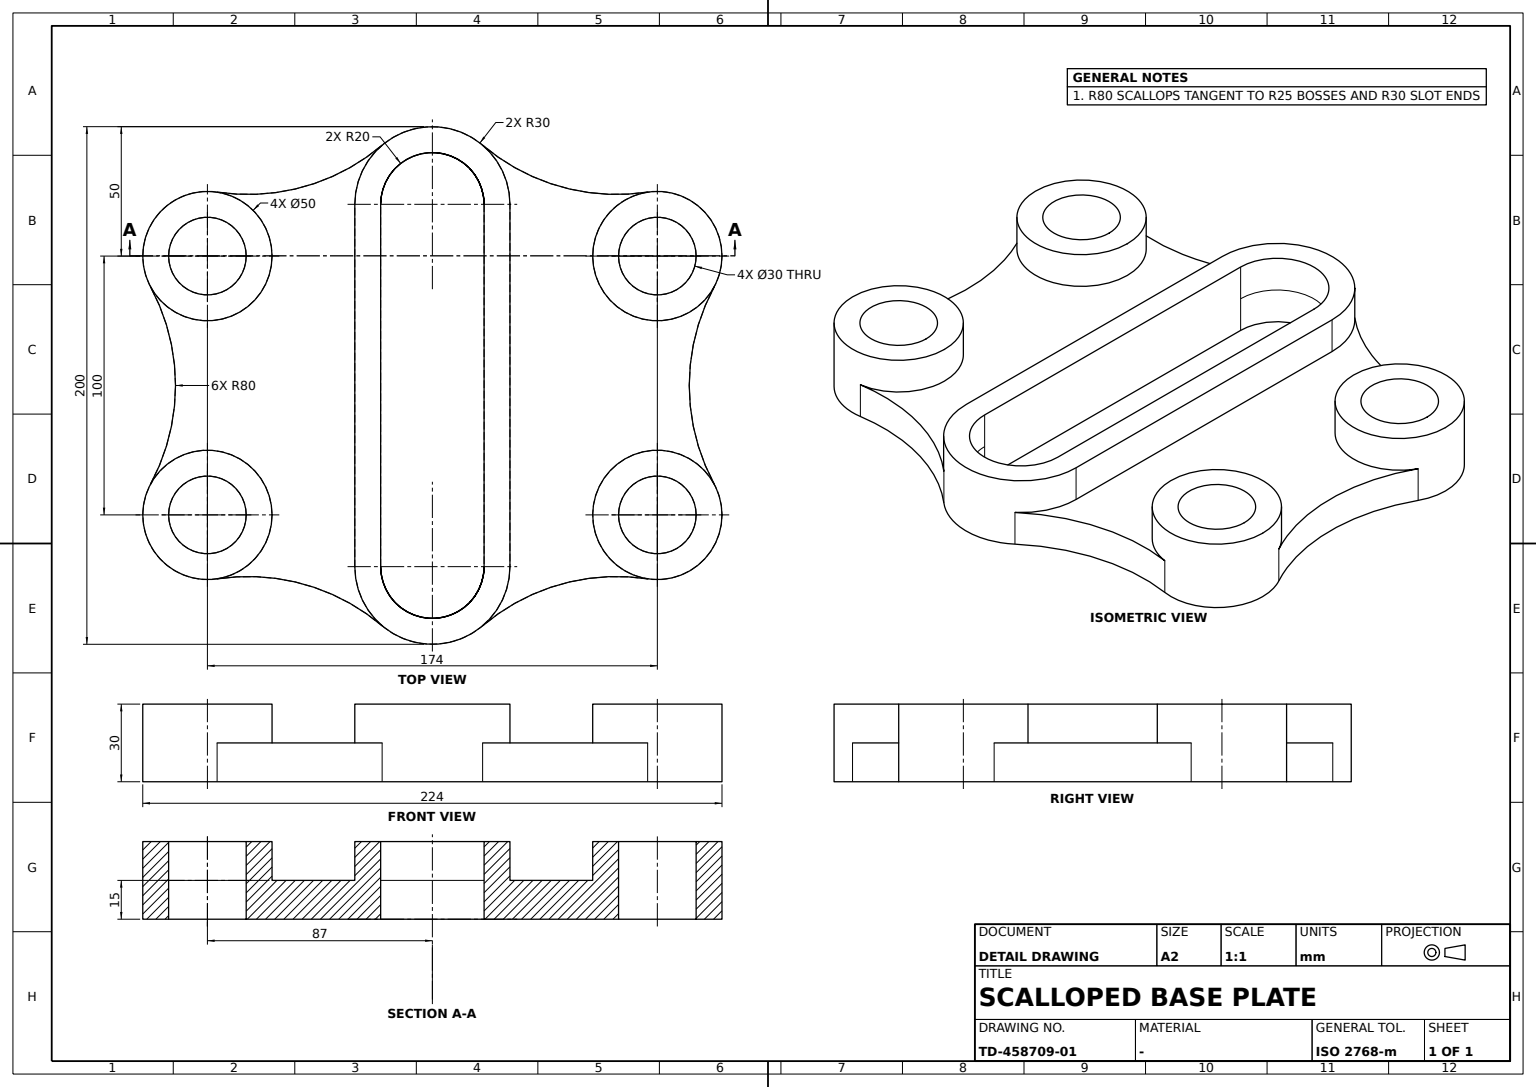
ISO-10303-21;
HEADER;
FILE_DESCRIPTION((''),'2;1');
FILE_NAME('','',(''),(''),'','','');
FILE_SCHEMA(('AUTOMOTIVE_DESIGN'));
ENDSEC;
DATA;
#1=APPLICATION_CONTEXT('');
#2=PRODUCT_CONTEXT('',#1,'mechanical');
#3=PRODUCT('','','',(#2));
#4=PRODUCT_DEFINITION_FORMATION('','',#3);
#5=PRODUCT_DEFINITION_CONTEXT('',#1,'design');
#6=PRODUCT_DEFINITION('','',#4,#5);
#7=PRODUCT_DEFINITION_SHAPE('','',#6);
#8=(LENGTH_UNIT()NAMED_UNIT(*)SI_UNIT(.MILLI.,.METRE.));
#9=(NAMED_UNIT(*)PLANE_ANGLE_UNIT()SI_UNIT($,.RADIAN.));
#10=(NAMED_UNIT(*)SI_UNIT($,.STERADIAN.)SOLID_ANGLE_UNIT());
#11=UNCERTAINTY_MEASURE_WITH_UNIT(LENGTH_MEASURE(0.005),#8,'distance_accuracy_value','');
#12=(GEOMETRIC_REPRESENTATION_CONTEXT(3)GLOBAL_UNCERTAINTY_ASSIGNED_CONTEXT((#11))GLOBAL_UNIT_ASSIGNED_CONTEXT((#8,#9,#10))REPRESENTATION_CONTEXT('',''));
#13=CARTESIAN_POINT('',(-20.,70.,0.));
#14=VERTEX_POINT('',#13);
#15=CARTESIAN_POINT('',(20.,70.,0.));
#16=VERTEX_POINT('',#15);
#17=CARTESIAN_POINT('',(-20.,75.235987756,0.));
#18=CARTESIAN_POINT('',(-15.672232498,85.666277369,0.));
#19=CARTESIAN_POINT('',(0.,92.166861315,0.));
#20=CARTESIAN_POINT('',(15.672232498,85.666277369,0.));
#21=CARTESIAN_POINT('',(20.,75.235987756,0.));
#22=B_SPLINE_CURVE_WITH_KNOTS('',3,(#13,#17,#18,#19,#20,#21,#15),.UNSPECIFIED.,.F.,.F.,(4,1,1,1,4),(0.,15.707963268,31.415926536,47.123889804,62.831853072),.UNSPECIFIED.);
#23=EDGE_CURVE('',#14,#16,#22,.T.);
#24=ORIENTED_EDGE('',*,*,#23,.F.);
#25=CARTESIAN_POINT('',(-20.,70.,-15.));
#26=VERTEX_POINT('',#25);
#27=DIRECTION('',(0.,0.,1.));
#28=VECTOR('',#27,1000.);
#29=LINE('',#13,#28);
#30=EDGE_CURVE('',#14,#26,#29,.F.);
#31=ORIENTED_EDGE('',*,*,#30,.T.);
#32=CARTESIAN_POINT('',(20.,70.,-15.));
#33=VERTEX_POINT('',#32);
#34=CARTESIAN_POINT('',(20.,75.235987756,-15.));
#35=CARTESIAN_POINT('',(15.672232498,85.666277369,-15.));
#36=CARTESIAN_POINT('',(0.,92.166861315,-15.));
#37=CARTESIAN_POINT('',(-15.672232498,85.666277369,-15.));
#38=CARTESIAN_POINT('',(-20.,75.235987756,-15.));
#39=B_SPLINE_CURVE_WITH_KNOTS('',3,(#32,#34,#35,#36,#37,#38,#25),.UNSPECIFIED.,.F.,.F.,(4,1,1,1,4),(140.,155.707963268,171.415926536,187.123889804,202.831853072),.UNSPECIFIED.);
#40=EDGE_CURVE('',#26,#33,#39,.F.);
#41=ORIENTED_EDGE('',*,*,#40,.T.);
#42=LINE('',#15,#28);
#43=EDGE_CURVE('',#16,#33,#42,.F.);
#44=ORIENTED_EDGE('',*,*,#43,.F.);
#45=EDGE_LOOP('',(#24,#31,#41,#44));
#46=FACE_BOUND('',#45,.T.);
#47=B_SPLINE_SURFACE_WITH_KNOTS('',3,1,((#13,#25),(#17,#38),(#18,#37),(#19,#36),(#20,#35),(#21,#34),(#15,#32)),.SURF_OF_LINEAR_EXTRUSION.,.F.,.F.,.F.,(4,1,1,1,4),(2,2),(0.,0.016,0.032,0.048,0.064),(0.,1.),.UNSPECIFIED.);
#48=ADVANCED_FACE('',(#46),#47,.F.);
#49=CARTESIAN_POINT('',(19.430163575,92.857575187,-15.));
#50=VERTEX_POINT('',#49);
#51=CARTESIAN_POINT('',(-19.430163575,92.857575187,-15.));
#52=VERTEX_POINT('',#51);
#53=CARTESIAN_POINT('',(0.,70.,-15.));
#54=DIRECTION('',(1.,0.,0.));
#55=AXIS2_PLACEMENT_3D('',#53,#27,#54);
#56=CIRCLE('',#55,30.);
#57=EDGE_CURVE('',#50,#52,#56,.T.);
#58=ORIENTED_EDGE('',*,*,#57,.T.);
#59=CARTESIAN_POINT('',(-19.430163575,92.857575187,0.));
#60=VERTEX_POINT('',#59);
#61=CARTESIAN_POINT('',(-19.430163575,92.857575187,-7.5));
#62=LINE('',#61,#28);
#63=EDGE_CURVE('',#60,#52,#62,.F.);
#64=ORIENTED_EDGE('',*,*,#63,.F.);
#65=CARTESIAN_POINT('',(-30.,70.,0.));
#66=VERTEX_POINT('',#65);
#67=CARTESIAN_POINT('',(0.,70.,0.));
#68=AXIS2_PLACEMENT_3D('',#67,#27,#54);
#69=CIRCLE('',#68,30.);
#70=EDGE_CURVE('',#60,#66,#69,.T.);
#71=ORIENTED_EDGE('',*,*,#70,.T.);
#72=CARTESIAN_POINT('',(-30.,70.,15.));
#73=VERTEX_POINT('',#72);
#74=CARTESIAN_POINT('',(-30.,70.,-7.5));
#75=LINE('',#74,#28);
#76=EDGE_CURVE('',#66,#73,#75,.T.);
#77=ORIENTED_EDGE('',*,*,#76,.T.);
#78=CARTESIAN_POINT('',(30.,70.,15.));
#79=VERTEX_POINT('',#78);
#80=CARTESIAN_POINT('',(0.,70.,15.));
#81=AXIS2_PLACEMENT_3D('',#80,#27,#54);
#82=CIRCLE('',#81,30.);
#83=EDGE_CURVE('',#79,#73,#82,.T.);
#84=ORIENTED_EDGE('',*,*,#83,.F.);
#85=CARTESIAN_POINT('',(30.,70.,0.));
#86=VERTEX_POINT('',#85);
#87=CARTESIAN_POINT('',(30.,70.,-7.5));
#88=LINE('',#87,#28);
#89=EDGE_CURVE('',#86,#79,#88,.T.);
#90=ORIENTED_EDGE('',*,*,#89,.F.);
#91=CARTESIAN_POINT('',(19.430163575,92.857575187,0.));
#92=VERTEX_POINT('',#91);
#93=EDGE_CURVE('',#86,#92,#69,.T.);
#94=ORIENTED_EDGE('',*,*,#93,.T.);
#95=CARTESIAN_POINT('',(19.430163575,92.857575187,-7.5));
#96=LINE('',#95,#28);
#97=EDGE_CURVE('',#92,#50,#96,.F.);
#98=ORIENTED_EDGE('',*,*,#97,.T.);
#99=EDGE_LOOP('',(#58,#64,#71,#77,#84,#90,#94,#98));
#100=FACE_BOUND('',#99,.T.);
#101=CARTESIAN_POINT('',(0.,70.,-7.5));
#102=AXIS2_PLACEMENT_3D('',#101,#27,#54);
#103=CYLINDRICAL_SURFACE('',#102,30.);
#104=ADVANCED_FACE('',(#100),#103,.T.);
#105=ORIENTED_EDGE('',*,*,#30,.F.);
#106=CARTESIAN_POINT('',(-20.,70.,15.));
#107=VERTEX_POINT('',#106);
#108=CARTESIAN_POINT('',(-20.,70.,7.5));
#109=LINE('',#108,#28);
#110=EDGE_CURVE('',#14,#107,#109,.T.);
#111=ORIENTED_EDGE('',*,*,#110,.T.);
#112=CARTESIAN_POINT('',(-20.,-70.,15.));
#113=VERTEX_POINT('',#112);
#114=CARTESIAN_POINT('',(-20.,0.,15.));
#115=DIRECTION('',(0.,1.,0.));
#116=VECTOR('',#115,1000.);
#117=LINE('',#114,#116);
#118=EDGE_CURVE('',#113,#107,#117,.T.);
#119=ORIENTED_EDGE('',*,*,#118,.F.);
#120=CARTESIAN_POINT('',(-20.,-70.,0.));
#121=VERTEX_POINT('',#120);
#122=CARTESIAN_POINT('',(-20.,-70.,7.5));
#123=LINE('',#122,#28);
#124=EDGE_CURVE('',#121,#113,#123,.T.);
#125=ORIENTED_EDGE('',*,*,#124,.F.);
#126=CARTESIAN_POINT('',(-20.,-70.,-15.));
#127=VERTEX_POINT('',#126);
#128=LINE('',#120,#28);
#129=EDGE_CURVE('',#121,#127,#128,.F.);
#130=ORIENTED_EDGE('',*,*,#129,.T.);
#131=CARTESIAN_POINT('',(-20.,0.,-15.));
#132=LINE('',#131,#116);
#133=EDGE_CURVE('',#127,#26,#132,.T.);
#134=ORIENTED_EDGE('',*,*,#133,.T.);
#135=EDGE_LOOP('',(#105,#111,#119,#125,#130,#134));
#136=FACE_BOUND('',#135,.T.);
#137=AXIS2_PLACEMENT_3D('',#120,#54,#115);
#138=PLANE('',#137);
#139=ADVANCED_FACE('',(#136),#138,.T.);
#140=CARTESIAN_POINT('',(83.248555502,-74.716930719,-15.));
#141=VERTEX_POINT('',#140);
#142=CARTESIAN_POINT('',(19.430163575,-92.857575187,-15.));
#143=VERTEX_POINT('',#142);
#144=CARTESIAN_POINT('',(71.243933108,-153.811109021,-15.));
#145=AXIS2_PLACEMENT_3D('',#144,#27,#54);
#146=CIRCLE('',#145,80.);
#147=EDGE_CURVE('',#141,#143,#146,.T.);
#148=ORIENTED_EDGE('',*,*,#147,.F.);
#149=CARTESIAN_POINT('',(83.2485555,-74.716930719,0.));
#150=VERTEX_POINT('',#149);
#151=CARTESIAN_POINT('',(83.248555502,-74.716930719,-7.499999979));
#152=LINE('',#151,#28);
#153=EDGE_CURVE('',#150,#141,#152,.F.);
#154=ORIENTED_EDGE('',*,*,#153,.F.);
#155=CARTESIAN_POINT('',(19.430163575,-92.857575187,0.));
#156=VERTEX_POINT('',#155);
#157=CARTESIAN_POINT('',(71.243933108,-153.811109021,0.));
#158=AXIS2_PLACEMENT_3D('',#157,#27,#54);
#159=CIRCLE('',#158,80.);
#160=EDGE_CURVE('',#150,#156,#159,.T.);
#161=ORIENTED_EDGE('',*,*,#160,.T.);
#162=CARTESIAN_POINT('',(19.430163575,-92.857575187,-7.5));
#163=LINE('',#162,#28);
#164=EDGE_CURVE('',#156,#143,#163,.F.);
#165=ORIENTED_EDGE('',*,*,#164,.T.);
#166=EDGE_LOOP('',(#148,#154,#161,#165));
#167=FACE_BOUND('',#166,.T.);
#168=CARTESIAN_POINT('',(71.243933108,-153.811109021,-7.5));
#169=AXIS2_PLACEMENT_3D('',#168,#27,#54);
#170=CYLINDRICAL_SURFACE('',#169,80.);
#171=ADVANCED_FACE('',(#167),#170,.F.);
#172=CARTESIAN_POINT('',(112.,-50.,15.));
#173=VERTEX_POINT('',#172);
#174=CARTESIAN_POINT('',(87.,-50.,15.));
#175=AXIS2_PLACEMENT_3D('',#174,#27,#54);
#176=CIRCLE('',#175,25.);
#177=EDGE_CURVE('',#173,#173,#176,.T.);
#178=ORIENTED_EDGE('',*,*,#177,.F.);
#179=EDGE_LOOP('',(#178));
#180=FACE_BOUND('',#179,.T.);
#181=CARTESIAN_POINT('',(108.983553943,-38.095238094,0.));
#182=VERTEX_POINT('',#181);
#183=CARTESIAN_POINT('',(87.,-50.,0.));
#184=AXIS2_PLACEMENT_3D('',#183,#27,#54);
#185=CIRCLE('',#184,25.);
#186=EDGE_CURVE('',#182,#150,#185,.T.);
#187=ORIENTED_EDGE('',*,*,#186,.T.);
#188=ORIENTED_EDGE('',*,*,#153,.T.);
#189=CARTESIAN_POINT('',(108.983553944,-38.095238095,-15.));
#190=VERTEX_POINT('',#189);
#191=CARTESIAN_POINT('',(87.,-50.,-15.));
#192=AXIS2_PLACEMENT_3D('',#191,#27,#54);
#193=CIRCLE('',#192,25.);
#194=EDGE_CURVE('',#141,#190,#193,.T.);
#195=ORIENTED_EDGE('',*,*,#194,.T.);
#196=CARTESIAN_POINT('',(108.983553944,-38.095238095,-7.499999979));
#197=LINE('',#196,#28);
#198=EDGE_CURVE('',#182,#190,#197,.F.);
#199=ORIENTED_EDGE('',*,*,#198,.F.);
#200=EDGE_LOOP('',(#187,#188,#195,#199));
#201=FACE_BOUND('',#200,.T.);
#202=CARTESIAN_POINT('',(87.,-50.,7.5));
#203=AXIS2_PLACEMENT_3D('',#202,#27,#54);
#204=CYLINDRICAL_SURFACE('',#203,25.);
#205=ADVANCED_FACE('',(#180,#201),#204,.T.);
#206=CARTESIAN_POINT('',(-19.430163575,-92.857575187,0.));
#207=VERTEX_POINT('',#206);
#208=CARTESIAN_POINT('',(-19.430163575,-92.857575187,-15.));
#209=VERTEX_POINT('',#208);
#210=CARTESIAN_POINT('',(-19.430163575,-92.857575187,-7.5));
#211=LINE('',#210,#28);
#212=EDGE_CURVE('',#207,#209,#211,.F.);
#213=ORIENTED_EDGE('',*,*,#212,.F.);
#214=CARTESIAN_POINT('',(-83.248555502,-74.716930719,0.));
#215=VERTEX_POINT('',#214);
#216=CARTESIAN_POINT('',(-71.243933108,-153.811109021,0.));
#217=AXIS2_PLACEMENT_3D('',#216,#27,#54);
#218=CIRCLE('',#217,80.);
#219=EDGE_CURVE('',#207,#215,#218,.T.);
#220=ORIENTED_EDGE('',*,*,#219,.T.);
#221=CARTESIAN_POINT('',(-83.248555502,-74.716930719,-15.));
#222=VERTEX_POINT('',#221);
#223=CARTESIAN_POINT('',(-83.248555502,-74.716930719,-7.5));
#224=LINE('',#223,#28);
#225=EDGE_CURVE('',#215,#222,#224,.F.);
#226=ORIENTED_EDGE('',*,*,#225,.T.);
#227=CARTESIAN_POINT('',(-71.243933108,-153.811109021,-15.));
#228=AXIS2_PLACEMENT_3D('',#227,#27,#54);
#229=CIRCLE('',#228,80.);
#230=EDGE_CURVE('',#209,#222,#229,.T.);
#231=ORIENTED_EDGE('',*,*,#230,.F.);
#232=EDGE_LOOP('',(#213,#220,#226,#231));
#233=FACE_BOUND('',#232,.T.);
#234=CARTESIAN_POINT('',(-71.243933108,-153.811109021,-7.5));
#235=AXIS2_PLACEMENT_3D('',#234,#27,#54);
#236=CYLINDRICAL_SURFACE('',#235,80.);
#237=ADVANCED_FACE('',(#233),#236,.F.);
#238=ORIENTED_EDGE('',*,*,#129,.F.);
#239=CARTESIAN_POINT('',(20.,-70.,0.));
#240=VERTEX_POINT('',#239);
#241=CARTESIAN_POINT('',(20.,-75.235987756,0.));
#242=CARTESIAN_POINT('',(15.672232498,-85.666277369,0.));
#243=CARTESIAN_POINT('',(0.,-92.166861315,0.));
#244=CARTESIAN_POINT('',(-15.672232498,-85.666277369,0.));
#245=CARTESIAN_POINT('',(-20.,-75.235987756,0.));
#246=B_SPLINE_CURVE_WITH_KNOTS('',3,(#239,#241,#242,#243,#244,#245,#120),.UNSPECIFIED.,.F.,.F.,(4,1,1,1,4),(62.831853072,78.53981634,94.247779608,109.955742876,125.663706144),.UNSPECIFIED.);
#247=EDGE_CURVE('',#240,#121,#246,.T.);
#248=ORIENTED_EDGE('',*,*,#247,.F.);
#249=CARTESIAN_POINT('',(20.,-70.,-15.));
#250=VERTEX_POINT('',#249);
#251=LINE('',#239,#28);
#252=EDGE_CURVE('',#240,#250,#251,.F.);
#253=ORIENTED_EDGE('',*,*,#252,.T.);
#254=CARTESIAN_POINT('',(-20.,-75.235987756,-15.));
#255=CARTESIAN_POINT('',(-15.672232498,-85.666277369,-15.));
#256=CARTESIAN_POINT('',(0.,-92.166861315,-15.));
#257=CARTESIAN_POINT('',(15.672232498,-85.666277369,-15.));
#258=CARTESIAN_POINT('',(20.,-75.235987756,-15.));
#259=B_SPLINE_CURVE_WITH_KNOTS('',3,(#126,#254,#255,#256,#257,#258,#249),.UNSPECIFIED.,.F.,.F.,(4,1,1,1,4),(342.831853072,358.53981634,374.247779608,389.955742876,405.663706144),.UNSPECIFIED.);
#260=EDGE_CURVE('',#250,#127,#259,.F.);
#261=ORIENTED_EDGE('',*,*,#260,.T.);
#262=EDGE_LOOP('',(#238,#248,#253,#261));
#263=FACE_BOUND('',#262,.T.);
#264=B_SPLINE_SURFACE_WITH_KNOTS('',3,1,((#239,#249),(#241,#258),(#242,#257),(#243,#256),(#244,#255),(#245,#254),(#120,#126)),.SURF_OF_LINEAR_EXTRUSION.,.F.,.F.,.F.,(4,1,1,1,4),(2,2),(0.,0.016,0.032,0.048,0.064),(0.,1.),.UNSPECIFIED.);
#265=ADVANCED_FACE('',(#263),#264,.F.);
#266=ORIENTED_EDGE('',*,*,#23,.T.);
#267=CARTESIAN_POINT('',(20.,70.,15.));
#268=VERTEX_POINT('',#267);
#269=CARTESIAN_POINT('',(20.,70.,7.5));
#270=LINE('',#269,#28);
#271=EDGE_CURVE('',#16,#268,#270,.T.);
#272=ORIENTED_EDGE('',*,*,#271,.T.);
#273=CIRCLE('',#81,20.);
#274=EDGE_CURVE('',#268,#107,#273,.T.);
#275=ORIENTED_EDGE('',*,*,#274,.T.);
#276=ORIENTED_EDGE('',*,*,#110,.F.);
#277=EDGE_LOOP('',(#266,#272,#275,#276));
#278=FACE_BOUND('',#277,.T.);
#279=CARTESIAN_POINT('',(0.,70.,7.5));
#280=AXIS2_PLACEMENT_3D('',#279,#27,#54);
#281=CYLINDRICAL_SURFACE('',#280,20.);
#282=ADVANCED_FACE('',(#278),#281,.F.);
#283=CARTESIAN_POINT('',(-62.,50.,15.));
#284=VERTEX_POINT('',#283);
#285=CARTESIAN_POINT('',(-87.,50.,15.));
#286=AXIS2_PLACEMENT_3D('',#285,#27,#54);
#287=CIRCLE('',#286,25.);
#288=EDGE_CURVE('',#284,#284,#287,.T.);
#289=ORIENTED_EDGE('',*,*,#288,.T.);
#290=EDGE_LOOP('',(#289));
#291=FACE_BOUND('',#290,.T.);
#292=CARTESIAN_POINT('',(-72.,50.,15.));
#293=VERTEX_POINT('',#292);
#294=CIRCLE('',#286,15.);
#295=EDGE_CURVE('',#293,#293,#294,.T.);
#296=ORIENTED_EDGE('',*,*,#295,.F.);
#297=EDGE_LOOP('',(#296));
#298=FACE_BOUND('',#297,.T.);
#299=CARTESIAN_POINT('',(0.,0.,15.));
#300=AXIS2_PLACEMENT_3D('',#299,#27,#54);
#301=PLANE('',#300);
#302=ADVANCED_FACE('',(#291,#298),#301,.T.);
#303=ORIENTED_EDGE('',*,*,#260,.F.);
#304=CARTESIAN_POINT('',(20.,0.,-15.));
#305=DIRECTION('',(0.,-1.,0.));
#306=VECTOR('',#305,1000.);
#307=LINE('',#304,#306);
#308=EDGE_CURVE('',#33,#250,#307,.T.);
#309=ORIENTED_EDGE('',*,*,#308,.F.);
#310=ORIENTED_EDGE('',*,*,#40,.F.);
#311=ORIENTED_EDGE('',*,*,#133,.F.);
#312=EDGE_LOOP('',(#303,#309,#310,#311));
#313=FACE_BOUND('',#312,.T.);
#314=CARTESIAN_POINT('',(83.248555502,74.716930719,-15.));
#315=VERTEX_POINT('',#314);
#316=CARTESIAN_POINT('',(71.243933108,153.811109021,-15.));
#317=AXIS2_PLACEMENT_3D('',#316,#27,#54);
#318=CIRCLE('',#317,80.);
#319=EDGE_CURVE('',#50,#315,#318,.T.);
#320=ORIENTED_EDGE('',*,*,#319,.T.);
#321=CARTESIAN_POINT('',(108.983553944,38.095238095,-15.));
#322=VERTEX_POINT('',#321);
#323=CARTESIAN_POINT('',(87.,50.,-15.));
#324=AXIS2_PLACEMENT_3D('',#323,#27,#54);
#325=CIRCLE('',#324,25.);
#326=EDGE_CURVE('',#322,#315,#325,.T.);
#327=ORIENTED_EDGE('',*,*,#326,.F.);
#328=CARTESIAN_POINT('',(179.330926563,0.,-15.));
#329=AXIS2_PLACEMENT_3D('',#328,#27,#54);
#330=CIRCLE('',#329,80.);
#331=EDGE_CURVE('',#322,#190,#330,.T.);
#332=ORIENTED_EDGE('',*,*,#331,.T.);
#333=ORIENTED_EDGE('',*,*,#194,.F.);
#334=ORIENTED_EDGE('',*,*,#147,.T.);
#335=CARTESIAN_POINT('',(0.,-70.,-15.));
#336=AXIS2_PLACEMENT_3D('',#335,#27,#54);
#337=CIRCLE('',#336,30.);
#338=EDGE_CURVE('',#209,#143,#337,.T.);
#339=ORIENTED_EDGE('',*,*,#338,.F.);
#340=ORIENTED_EDGE('',*,*,#230,.T.);
#341=CARTESIAN_POINT('',(-108.983553944,-38.095238095,-15.));
#342=VERTEX_POINT('',#341);
#343=CARTESIAN_POINT('',(-87.,-50.,-15.));
#344=AXIS2_PLACEMENT_3D('',#343,#27,#54);
#345=CIRCLE('',#344,25.);
#346=EDGE_CURVE('',#342,#222,#345,.T.);
#347=ORIENTED_EDGE('',*,*,#346,.F.);
#348=CARTESIAN_POINT('',(-108.983553944,38.095238095,-15.));
#349=VERTEX_POINT('',#348);
#350=CARTESIAN_POINT('',(-179.330926563,0.,-15.));
#351=AXIS2_PLACEMENT_3D('',#350,#27,#54);
#352=CIRCLE('',#351,80.);
#353=EDGE_CURVE('',#342,#349,#352,.T.);
#354=ORIENTED_EDGE('',*,*,#353,.T.);
#355=CARTESIAN_POINT('',(-83.248555502,74.716930719,-15.));
#356=VERTEX_POINT('',#355);
#357=CARTESIAN_POINT('',(-87.,50.,-15.));
#358=AXIS2_PLACEMENT_3D('',#357,#27,#54);
#359=CIRCLE('',#358,25.);
#360=EDGE_CURVE('',#356,#349,#359,.T.);
#361=ORIENTED_EDGE('',*,*,#360,.F.);
#362=CARTESIAN_POINT('',(-71.243933108,153.811109021,-15.));
#363=AXIS2_PLACEMENT_3D('',#362,#27,#54);
#364=CIRCLE('',#363,80.);
#365=EDGE_CURVE('',#356,#52,#364,.T.);
#366=ORIENTED_EDGE('',*,*,#365,.T.);
#367=ORIENTED_EDGE('',*,*,#57,.F.);
#368=EDGE_LOOP('',(#320,#327,#332,#333,#334,#339,#340,#347,#354,#361,#366,#367));
#369=FACE_BOUND('',#368,.T.);
#370=CARTESIAN_POINT('',(-72.,-50.,-15.));
#371=VERTEX_POINT('',#370);
#372=CIRCLE('',#344,15.);
#373=EDGE_CURVE('',#371,#371,#372,.T.);
#374=ORIENTED_EDGE('',*,*,#373,.T.);
#375=EDGE_LOOP('',(#374));
#376=FACE_BOUND('',#375,.T.);
#377=CARTESIAN_POINT('',(102.,50.,-15.));
#378=VERTEX_POINT('',#377);
#379=CIRCLE('',#324,15.);
#380=EDGE_CURVE('',#378,#378,#379,.T.);
#381=ORIENTED_EDGE('',*,*,#380,.T.);
#382=EDGE_LOOP('',(#381));
#383=FACE_BOUND('',#382,.T.);
#384=CARTESIAN_POINT('',(-72.,50.,-15.));
#385=VERTEX_POINT('',#384);
#386=CIRCLE('',#358,15.);
#387=EDGE_CURVE('',#385,#385,#386,.T.);
#388=ORIENTED_EDGE('',*,*,#387,.T.);
#389=EDGE_LOOP('',(#388));
#390=FACE_BOUND('',#389,.T.);
#391=CARTESIAN_POINT('',(102.,-50.,-15.));
#392=VERTEX_POINT('',#391);
#393=CIRCLE('',#192,15.);
#394=EDGE_CURVE('',#392,#392,#393,.T.);
#395=ORIENTED_EDGE('',*,*,#394,.T.);
#396=EDGE_LOOP('',(#395));
#397=FACE_BOUND('',#396,.T.);
#398=CARTESIAN_POINT('',(0.,0.,-15.));
#399=AXIS2_PLACEMENT_3D('',#398,#27,#54);
#400=PLANE('',#399);
#401=ADVANCED_FACE('',(#313,#369,#376,#383,#390,#397),#400,.F.);
#402=ORIENTED_EDGE('',*,*,#76,.F.);
#403=CARTESIAN_POINT('',(-30.,-70.,0.));
#404=VERTEX_POINT('',#403);
#405=CARTESIAN_POINT('',(-30.,0.,0.));
#406=LINE('',#405,#116);
#407=EDGE_CURVE('',#404,#66,#406,.T.);
#408=ORIENTED_EDGE('',*,*,#407,.F.);
#409=CARTESIAN_POINT('',(-30.,-70.,15.));
#410=VERTEX_POINT('',#409);
#411=CARTESIAN_POINT('',(-30.,-70.,-7.5));
#412=LINE('',#411,#28);
#413=EDGE_CURVE('',#404,#410,#412,.T.);
#414=ORIENTED_EDGE('',*,*,#413,.T.);
#415=CARTESIAN_POINT('',(-30.,0.,15.));
#416=LINE('',#415,#116);
#417=EDGE_CURVE('',#410,#73,#416,.T.);
#418=ORIENTED_EDGE('',*,*,#417,.T.);
#419=EDGE_LOOP('',(#402,#408,#414,#418));
#420=FACE_BOUND('',#419,.T.);
#421=AXIS2_PLACEMENT_3D('',#403,#54,#115);
#422=PLANE('',#421);
#423=ADVANCED_FACE('',(#420),#422,.F.);
#424=CARTESIAN_POINT('',(30.,-70.,0.));
#425=VERTEX_POINT('',#424);
#426=CARTESIAN_POINT('',(0.,-70.,0.));
#427=AXIS2_PLACEMENT_3D('',#426,#27,#54);
#428=CIRCLE('',#427,30.);
#429=EDGE_CURVE('',#156,#425,#428,.T.);
#430=ORIENTED_EDGE('',*,*,#429,.F.);
#431=ORIENTED_EDGE('',*,*,#160,.F.);
#432=ORIENTED_EDGE('',*,*,#186,.F.);
#433=CARTESIAN_POINT('',(108.983553943,38.095238094,0.));
#434=VERTEX_POINT('',#433);
#435=CARTESIAN_POINT('',(179.330926563,0.,0.));
#436=AXIS2_PLACEMENT_3D('',#435,#27,#54);
#437=CIRCLE('',#436,80.);
#438=EDGE_CURVE('',#434,#182,#437,.T.);
#439=ORIENTED_EDGE('',*,*,#438,.F.);
#440=CARTESIAN_POINT('',(83.2485555,74.716930719,0.));
#441=VERTEX_POINT('',#440);
#442=CARTESIAN_POINT('',(87.,50.,0.));
#443=AXIS2_PLACEMENT_3D('',#442,#27,#54);
#444=CIRCLE('',#443,25.);
#445=EDGE_CURVE('',#441,#434,#444,.T.);
#446=ORIENTED_EDGE('',*,*,#445,.F.);
#447=CARTESIAN_POINT('',(71.243933108,153.811109021,0.));
#448=AXIS2_PLACEMENT_3D('',#447,#27,#54);
#449=CIRCLE('',#448,80.);
#450=EDGE_CURVE('',#92,#441,#449,.T.);
#451=ORIENTED_EDGE('',*,*,#450,.F.);
#452=ORIENTED_EDGE('',*,*,#93,.F.);
#453=CARTESIAN_POINT('',(30.,0.,0.));
#454=LINE('',#453,#306);
#455=EDGE_CURVE('',#86,#425,#454,.T.);
#456=ORIENTED_EDGE('',*,*,#455,.T.);
#457=EDGE_LOOP('',(#430,#431,#432,#439,#446,#451,#452,#456));
#458=FACE_BOUND('',#457,.T.);
#459=CARTESIAN_POINT('',(0.,0.,0.));
#460=AXIS2_PLACEMENT_3D('',#459,#27,#54);
#461=PLANE('',#460);
#462=ADVANCED_FACE('',(#458),#461,.T.);
#463=CARTESIAN_POINT('',(-108.983553944,-38.095238095,0.));
#464=VERTEX_POINT('',#463);
#465=CARTESIAN_POINT('',(-108.983553944,38.095238095,0.));
#466=VERTEX_POINT('',#465);
#467=CARTESIAN_POINT('',(-179.330926563,0.,0.));
#468=AXIS2_PLACEMENT_3D('',#467,#27,#54);
#469=CIRCLE('',#468,80.);
#470=EDGE_CURVE('',#464,#466,#469,.T.);
#471=ORIENTED_EDGE('',*,*,#470,.T.);
#472=CARTESIAN_POINT('',(-108.983553944,38.095238095,-7.5));
#473=LINE('',#472,#28);
#474=EDGE_CURVE('',#466,#349,#473,.F.);
#475=ORIENTED_EDGE('',*,*,#474,.T.);
#476=ORIENTED_EDGE('',*,*,#353,.F.);
#477=CARTESIAN_POINT('',(-108.983553944,-38.095238095,-7.5));
#478=LINE('',#477,#28);
#479=EDGE_CURVE('',#464,#342,#478,.F.);
#480=ORIENTED_EDGE('',*,*,#479,.F.);
#481=EDGE_LOOP('',(#471,#475,#476,#480));
#482=FACE_BOUND('',#481,.T.);
#483=CARTESIAN_POINT('',(-179.330926563,0.,-7.5));
#484=AXIS2_PLACEMENT_3D('',#483,#27,#54);
#485=CYLINDRICAL_SURFACE('',#484,80.);
#486=ADVANCED_FACE('',(#482),#485,.F.);
#487=ORIENTED_EDGE('',*,*,#288,.F.);
#488=EDGE_LOOP('',(#487));
#489=FACE_BOUND('',#488,.T.);
#490=ORIENTED_EDGE('',*,*,#474,.F.);
#491=CARTESIAN_POINT('',(-83.248555502,74.716930719,0.));
#492=VERTEX_POINT('',#491);
#493=CARTESIAN_POINT('',(-87.,50.,0.));
#494=AXIS2_PLACEMENT_3D('',#493,#27,#54);
#495=CIRCLE('',#494,25.);
#496=EDGE_CURVE('',#466,#492,#495,.T.);
#497=ORIENTED_EDGE('',*,*,#496,.T.);
#498=CARTESIAN_POINT('',(-83.248555502,74.716930719,-7.5));
#499=LINE('',#498,#28);
#500=EDGE_CURVE('',#492,#356,#499,.F.);
#501=ORIENTED_EDGE('',*,*,#500,.T.);
#502=ORIENTED_EDGE('',*,*,#360,.T.);
#503=EDGE_LOOP('',(#490,#497,#501,#502));
#504=FACE_BOUND('',#503,.T.);
#505=CARTESIAN_POINT('',(-87.,50.,7.5));
#506=AXIS2_PLACEMENT_3D('',#505,#27,#54);
#507=CYLINDRICAL_SURFACE('',#506,25.);
#508=ADVANCED_FACE('',(#489,#504),#507,.T.);
#509=CARTESIAN_POINT('',(112.,50.,15.));
#510=VERTEX_POINT('',#509);
#511=CARTESIAN_POINT('',(87.,50.,15.));
#512=AXIS2_PLACEMENT_3D('',#511,#27,#54);
#513=CIRCLE('',#512,25.);
#514=EDGE_CURVE('',#510,#510,#513,.T.);
#515=ORIENTED_EDGE('',*,*,#514,.T.);
#516=EDGE_LOOP('',(#515));
#517=FACE_BOUND('',#516,.T.);
#518=CARTESIAN_POINT('',(102.,50.,15.));
#519=VERTEX_POINT('',#518);
#520=CIRCLE('',#512,15.);
#521=EDGE_CURVE('',#519,#519,#520,.T.);
#522=ORIENTED_EDGE('',*,*,#521,.F.);
#523=EDGE_LOOP('',(#522));
#524=FACE_BOUND('',#523,.T.);
#525=ADVANCED_FACE('',(#517,#524),#301,.T.);
#526=CARTESIAN_POINT('',(83.248555502,74.716930719,-7.499999979));
#527=LINE('',#526,#28);
#528=EDGE_CURVE('',#441,#315,#527,.F.);
#529=ORIENTED_EDGE('',*,*,#528,.T.);
#530=ORIENTED_EDGE('',*,*,#319,.F.);
#531=ORIENTED_EDGE('',*,*,#97,.F.);
#532=ORIENTED_EDGE('',*,*,#450,.T.);
#533=EDGE_LOOP('',(#529,#530,#531,#532));
#534=FACE_BOUND('',#533,.T.);
#535=CARTESIAN_POINT('',(71.243933108,153.811109021,-7.5));
#536=AXIS2_PLACEMENT_3D('',#535,#27,#54);
#537=CYLINDRICAL_SURFACE('',#536,80.);
#538=ADVANCED_FACE('',(#534),#537,.F.);
#539=CARTESIAN_POINT('',(-62.,-50.,15.));
#540=VERTEX_POINT('',#539);
#541=CARTESIAN_POINT('',(-87.,-50.,15.));
#542=AXIS2_PLACEMENT_3D('',#541,#27,#54);
#543=CIRCLE('',#542,25.);
#544=EDGE_CURVE('',#540,#540,#543,.T.);
#545=ORIENTED_EDGE('',*,*,#544,.T.);
#546=EDGE_LOOP('',(#545));
#547=FACE_BOUND('',#546,.T.);
#548=CARTESIAN_POINT('',(-72.,-50.,15.));
#549=VERTEX_POINT('',#548);
#550=CIRCLE('',#542,15.);
#551=EDGE_CURVE('',#549,#549,#550,.T.);
#552=ORIENTED_EDGE('',*,*,#551,.F.);
#553=EDGE_LOOP('',(#552));
#554=FACE_BOUND('',#553,.T.);
#555=ADVANCED_FACE('',(#547,#554),#301,.T.);
#556=ORIENTED_EDGE('',*,*,#394,.F.);
#557=EDGE_LOOP('',(#556));
#558=FACE_BOUND('',#557,.T.);
#559=CARTESIAN_POINT('',(102.,-50.,15.));
#560=VERTEX_POINT('',#559);
#561=CIRCLE('',#175,15.);
#562=EDGE_CURVE('',#560,#560,#561,.T.);
#563=ORIENTED_EDGE('',*,*,#562,.T.);
#564=EDGE_LOOP('',(#563));
#565=FACE_BOUND('',#564,.T.);
#566=CARTESIAN_POINT('',(87.,-50.,-7.5));
#567=AXIS2_PLACEMENT_3D('',#566,#27,#54);
#568=CYLINDRICAL_SURFACE('',#567,15.);
#569=ADVANCED_FACE('',(#558,#565),#568,.F.);
#570=ORIENTED_EDGE('',*,*,#413,.F.);
#571=EDGE_CURVE('',#404,#207,#428,.T.);
#572=ORIENTED_EDGE('',*,*,#571,.T.);
#573=ORIENTED_EDGE('',*,*,#212,.T.);
#574=ORIENTED_EDGE('',*,*,#338,.T.);
#575=ORIENTED_EDGE('',*,*,#164,.F.);
#576=ORIENTED_EDGE('',*,*,#429,.T.);
#577=CARTESIAN_POINT('',(30.,-70.,15.));
#578=VERTEX_POINT('',#577);
#579=CARTESIAN_POINT('',(30.,-70.,-7.5));
#580=LINE('',#579,#28);
#581=EDGE_CURVE('',#425,#578,#580,.T.);
#582=ORIENTED_EDGE('',*,*,#581,.T.);
#583=CARTESIAN_POINT('',(0.,-70.,15.));
#584=AXIS2_PLACEMENT_3D('',#583,#27,#54);
#585=CIRCLE('',#584,30.);
#586=EDGE_CURVE('',#410,#578,#585,.T.);
#587=ORIENTED_EDGE('',*,*,#586,.F.);
#588=EDGE_LOOP('',(#570,#572,#573,#574,#575,#576,#582,#587));
#589=FACE_BOUND('',#588,.T.);
#590=CARTESIAN_POINT('',(0.,-70.,-7.5));
#591=AXIS2_PLACEMENT_3D('',#590,#27,#54);
#592=CYLINDRICAL_SURFACE('',#591,30.);
#593=ADVANCED_FACE('',(#589),#592,.T.);
#594=ORIENTED_EDGE('',*,*,#387,.F.);
#595=EDGE_LOOP('',(#594));
#596=FACE_BOUND('',#595,.T.);
#597=ORIENTED_EDGE('',*,*,#295,.T.);
#598=EDGE_LOOP('',(#597));
#599=FACE_BOUND('',#598,.T.);
#600=CARTESIAN_POINT('',(-87.,50.,-7.5));
#601=AXIS2_PLACEMENT_3D('',#600,#27,#54);
#602=CYLINDRICAL_SURFACE('',#601,15.);
#603=ADVANCED_FACE('',(#596,#599),#602,.F.);
#604=ORIENTED_EDGE('',*,*,#521,.T.);
#605=EDGE_LOOP('',(#604));
#606=FACE_BOUND('',#605,.T.);
#607=ORIENTED_EDGE('',*,*,#380,.F.);
#608=EDGE_LOOP('',(#607));
#609=FACE_BOUND('',#608,.T.);
#610=CARTESIAN_POINT('',(87.,50.,-7.5));
#611=AXIS2_PLACEMENT_3D('',#610,#27,#54);
#612=CYLINDRICAL_SURFACE('',#611,15.);
#613=ADVANCED_FACE('',(#606,#609),#612,.F.);
#614=ORIENTED_EDGE('',*,*,#373,.F.);
#615=EDGE_LOOP('',(#614));
#616=FACE_BOUND('',#615,.T.);
#617=ORIENTED_EDGE('',*,*,#551,.T.);
#618=EDGE_LOOP('',(#617));
#619=FACE_BOUND('',#618,.T.);
#620=CARTESIAN_POINT('',(-87.,-50.,-7.5));
#621=AXIS2_PLACEMENT_3D('',#620,#27,#54);
#622=CYLINDRICAL_SURFACE('',#621,15.);
#623=ADVANCED_FACE('',(#616,#619),#622,.F.);
#624=CARTESIAN_POINT('',(108.983553944,38.095238095,-7.499999979));
#625=LINE('',#624,#28);
#626=EDGE_CURVE('',#434,#322,#625,.F.);
#627=ORIENTED_EDGE('',*,*,#626,.T.);
#628=ORIENTED_EDGE('',*,*,#326,.T.);
#629=ORIENTED_EDGE('',*,*,#528,.F.);
#630=ORIENTED_EDGE('',*,*,#445,.T.);
#631=EDGE_LOOP('',(#627,#628,#629,#630));
#632=FACE_BOUND('',#631,.T.);
#633=ORIENTED_EDGE('',*,*,#514,.F.);
#634=EDGE_LOOP('',(#633));
#635=FACE_BOUND('',#634,.T.);
#636=CARTESIAN_POINT('',(87.,50.,7.5));
#637=AXIS2_PLACEMENT_3D('',#636,#27,#54);
#638=CYLINDRICAL_SURFACE('',#637,25.);
#639=ADVANCED_FACE('',(#632,#635),#638,.T.);
#640=ORIENTED_EDGE('',*,*,#581,.F.);
#641=ORIENTED_EDGE('',*,*,#455,.F.);
#642=ORIENTED_EDGE('',*,*,#89,.T.);
#643=CARTESIAN_POINT('',(30.,0.,15.));
#644=LINE('',#643,#306);
#645=EDGE_CURVE('',#79,#578,#644,.T.);
#646=ORIENTED_EDGE('',*,*,#645,.T.);
#647=EDGE_LOOP('',(#640,#641,#642,#646));
#648=FACE_BOUND('',#647,.T.);
#649=DIRECTION('',(-1.,0.,0.));
#650=AXIS2_PLACEMENT_3D('',#85,#649,#305);
#651=PLANE('',#650);
#652=ADVANCED_FACE('',(#648),#651,.F.);
#653=ORIENTED_EDGE('',*,*,#479,.T.);
#654=ORIENTED_EDGE('',*,*,#346,.T.);
#655=ORIENTED_EDGE('',*,*,#225,.F.);
#656=CARTESIAN_POINT('',(-87.,-50.,0.));
#657=AXIS2_PLACEMENT_3D('',#656,#27,#54);
#658=CIRCLE('',#657,25.);
#659=EDGE_CURVE('',#215,#464,#658,.T.);
#660=ORIENTED_EDGE('',*,*,#659,.T.);
#661=EDGE_LOOP('',(#653,#654,#655,#660));
#662=FACE_BOUND('',#661,.T.);
#663=ORIENTED_EDGE('',*,*,#544,.F.);
#664=EDGE_LOOP('',(#663));
#665=FACE_BOUND('',#664,.T.);
#666=CARTESIAN_POINT('',(-87.,-50.,7.5));
#667=AXIS2_PLACEMENT_3D('',#666,#27,#54);
#668=CYLINDRICAL_SURFACE('',#667,25.);
#669=ADVANCED_FACE('',(#662,#665),#668,.T.);
#670=ORIENTED_EDGE('',*,*,#124,.T.);
#671=CARTESIAN_POINT('',(20.,-70.,15.));
#672=VERTEX_POINT('',#671);
#673=CIRCLE('',#584,20.);
#674=EDGE_CURVE('',#113,#672,#673,.T.);
#675=ORIENTED_EDGE('',*,*,#674,.T.);
#676=CARTESIAN_POINT('',(20.,-70.,7.5));
#677=LINE('',#676,#28);
#678=EDGE_CURVE('',#240,#672,#677,.T.);
#679=ORIENTED_EDGE('',*,*,#678,.F.);
#680=ORIENTED_EDGE('',*,*,#247,.T.);
#681=EDGE_LOOP('',(#670,#675,#679,#680));
#682=FACE_BOUND('',#681,.T.);
#683=CARTESIAN_POINT('',(0.,-70.,7.5));
#684=AXIS2_PLACEMENT_3D('',#683,#27,#54);
#685=CYLINDRICAL_SURFACE('',#684,20.);
#686=ADVANCED_FACE('',(#682),#685,.F.);
#687=ORIENTED_EDGE('',*,*,#252,.F.);
#688=ORIENTED_EDGE('',*,*,#678,.T.);
#689=CARTESIAN_POINT('',(20.,0.,15.));
#690=LINE('',#689,#306);
#691=EDGE_CURVE('',#268,#672,#690,.T.);
#692=ORIENTED_EDGE('',*,*,#691,.F.);
#693=ORIENTED_EDGE('',*,*,#271,.F.);
#694=ORIENTED_EDGE('',*,*,#43,.T.);
#695=ORIENTED_EDGE('',*,*,#308,.T.);
#696=EDGE_LOOP('',(#687,#688,#692,#693,#694,#695));
#697=FACE_BOUND('',#696,.T.);
#698=AXIS2_PLACEMENT_3D('',#15,#649,#305);
#699=PLANE('',#698);
#700=ADVANCED_FACE('',(#697),#699,.T.);
#701=ORIENTED_EDGE('',*,*,#198,.T.);
#702=ORIENTED_EDGE('',*,*,#331,.F.);
#703=ORIENTED_EDGE('',*,*,#626,.F.);
#704=ORIENTED_EDGE('',*,*,#438,.T.);
#705=EDGE_LOOP('',(#701,#702,#703,#704));
#706=FACE_BOUND('',#705,.T.);
#707=CARTESIAN_POINT('',(179.330926563,0.,-7.5));
#708=AXIS2_PLACEMENT_3D('',#707,#27,#54);
#709=CYLINDRICAL_SURFACE('',#708,80.);
#710=ADVANCED_FACE('',(#706),#709,.F.);
#711=CARTESIAN_POINT('',(-71.243933108,153.811109021,0.));
#712=AXIS2_PLACEMENT_3D('',#711,#27,#54);
#713=CIRCLE('',#712,80.);
#714=EDGE_CURVE('',#492,#60,#713,.T.);
#715=ORIENTED_EDGE('',*,*,#714,.F.);
#716=ORIENTED_EDGE('',*,*,#496,.F.);
#717=ORIENTED_EDGE('',*,*,#470,.F.);
#718=ORIENTED_EDGE('',*,*,#659,.F.);
#719=ORIENTED_EDGE('',*,*,#219,.F.);
#720=ORIENTED_EDGE('',*,*,#571,.F.);
#721=ORIENTED_EDGE('',*,*,#407,.T.);
#722=ORIENTED_EDGE('',*,*,#70,.F.);
#723=EDGE_LOOP('',(#715,#716,#717,#718,#719,#720,#721,#722));
#724=FACE_BOUND('',#723,.T.);
#725=ADVANCED_FACE('',(#724),#461,.T.);
#726=ORIENTED_EDGE('',*,*,#177,.T.);
#727=EDGE_LOOP('',(#726));
#728=FACE_BOUND('',#727,.T.);
#729=ORIENTED_EDGE('',*,*,#562,.F.);
#730=EDGE_LOOP('',(#729));
#731=FACE_BOUND('',#730,.T.);
#732=ADVANCED_FACE('',(#728,#731),#301,.T.);
#733=ORIENTED_EDGE('',*,*,#714,.T.);
#734=ORIENTED_EDGE('',*,*,#63,.T.);
#735=ORIENTED_EDGE('',*,*,#365,.F.);
#736=ORIENTED_EDGE('',*,*,#500,.F.);
#737=EDGE_LOOP('',(#733,#734,#735,#736));
#738=FACE_BOUND('',#737,.T.);
#739=CARTESIAN_POINT('',(-71.243933108,153.811109021,-7.5));
#740=AXIS2_PLACEMENT_3D('',#739,#27,#54);
#741=CYLINDRICAL_SURFACE('',#740,80.);
#742=ADVANCED_FACE('',(#738),#741,.F.);
#743=ORIENTED_EDGE('',*,*,#417,.F.);
#744=ORIENTED_EDGE('',*,*,#586,.T.);
#745=ORIENTED_EDGE('',*,*,#645,.F.);
#746=ORIENTED_EDGE('',*,*,#83,.T.);
#747=EDGE_LOOP('',(#743,#744,#745,#746));
#748=FACE_BOUND('',#747,.T.);
#749=ORIENTED_EDGE('',*,*,#118,.T.);
#750=ORIENTED_EDGE('',*,*,#274,.F.);
#751=ORIENTED_EDGE('',*,*,#691,.T.);
#752=ORIENTED_EDGE('',*,*,#674,.F.);
#753=EDGE_LOOP('',(#749,#750,#751,#752));
#754=FACE_BOUND('',#753,.T.);
#755=ADVANCED_FACE('',(#748,#754),#301,.T.);
#756=CLOSED_SHELL('',(#48,#104,#139,#171,#205,#237,#265,#282,#302,#401,#423,#462,#486,#508,#525,#538,#555,#569,#593,#603,#613,#623,#639,#652,#669,#686,#700,#710,#725,#732,#742,#755));
#757=MANIFOLD_SOLID_BREP('',#756);
#758=ADVANCED_BREP_SHAPE_REPRESENTATION('',(#757),#12);
#759=SHAPE_DEFINITION_REPRESENTATION(#7,#758);
ENDSEC;
END-ISO-10303-21;
